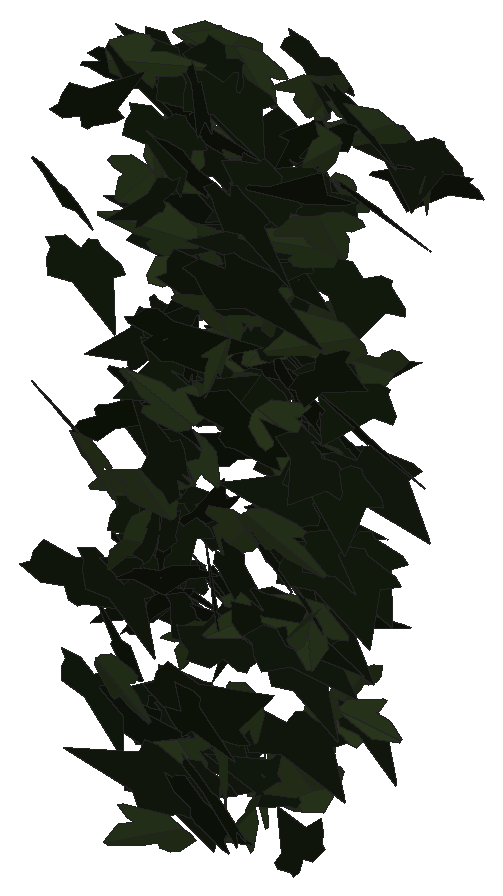
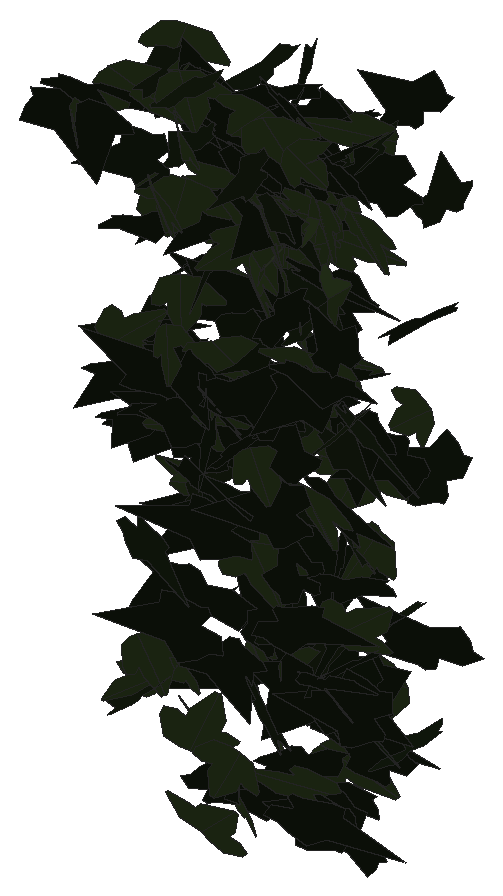
# SketchUp Ruby script. Lengths in millimetres.
U = 1.mm
M = Sketchup.active_model
def pt(a) = Geom::Point3d.new(a.map { |v| v * U })
def face(e, loops, mat)
  f = e.add_face(loops[0].map { |a| pt(a) })
  loops[1..].each { |l| e.add_face(l.map { |a| pt(a) }).erase! }
  f.material = f.back_material = mat if mat
  f
end
# faces: each face lists its corners as indices into pts; further lists are holes
def faces(e, pts, list, mat = nil) = list.each { |f| face(e, (f[0].is_a?(Array) ? f : [f]).map { |l| l.map { |i| pts[i] } }, mat) }
# xy, xz, yz: faces in a plane at the given z, y or x. An outline is a flat list of corners, or four numbers for a rectangle; further outlines are holes
def ring(l) = l.size == 4 ? [[l[0], l[1]], [l[2], l[1]], [l[2], l[3]], [l[0], l[3]]] : l.each_slice(2).to_a
def flat(e, list, mat, &to3) = list.each { |f| face(e, (f[0].is_a?(Array) ? f : [f]).map { |l| ring(l).map { |u, v| to3.(u, v) } }, mat) }
def xy(e, z, list, mat = nil) = flat(e, list, mat) { |x, y| [x, y, z] }
def xz(e, y, list, mat = nil) = flat(e, list, mat) { |x, z| [x, y, z] }
def yz(e, x, list, mat = nil) = flat(e, list, mat) { |y, z| [x, y, z] }
def lines(e, pts, list) = list.each { |a, b| e.add_line(pt(pts[a]), pt(pts[b])) }
# prism: a flat outline (further loops are holes) pulled along v
def prism(e, loops, v, mat = nil)
  f = face(e, loops, mat); d = Geom::Vector3d.new(v.map { |x| x * U })
  f.pushpull(f.normal.samedirection?(d) ? d.length : -d.length)
end
def box(e, o, s, mat = nil) = prism(e, [[o, [o[0] + s[0], o[1], o[2]], [o[0] + s[0], o[1] + s[1], o[2]], [o[0], o[1] + s[1], o[2]]]], [0, 0, s[2]], mat)
def at(x, y, z, deg = 0) = Geom::Transformation.translation(pt([x, y, z])) * Geom::Transformation.rotation(ORIGIN, Z_AXIS, deg.degrees)
def axes(o, x, y, z) = Geom::Transformation.new([*x, 0, *y, 0, *z, 0, *pt(o).to_a, 1])
def part(name) = M.definitions.add(name)
# library, detail: a bought-in or finely detailed component or shape, given as its bounding box
def library(name, o, s) = part(name).tap { |d| box(d.entities, o, s) }
def detail(e, o, s) = box(e.add_group.entities, o, s)
def put(e, d, t, mat = nil) = e.add_instance(d, t).tap { |i| i.material = mat if mat }
def group(e, t, mat = nil) = e.add_group.tap { |g| g.transformation = t; g.material = mat if mat }.entities
root = M.entities
M.materials.add("efeu1").color = [18, 25, 13]
M.materials.add("efeu2").color = [43, 57, 29]
c1 = part("ivyleaf_9")
p = [[39.1,54.8,31.7],[34.5,51.8,30.2],[-5.3,25.2,17.3],[-17.9,28.3,20.9],[-21.6,21.7,17],[-20.2,4.3,5.3],
  [-22.9,-0.3,2.5],[-17.1,-4,-0.6],[-2,-2.1,-1.2],[-0.7,-15.4,-10.1],[16.6,-22.3,-16.7],[21.1,-15.1,-12.5],
  [32.7,-10.7,-11],[46.1,-1.8,-6.6],[30.8,11.2,3.8]]
faces(c1.entities,p,[[0,1,2,3,4,5,6,7,8,9,10,11,12,13,14]],"efeu1")
c2 = part("ivyleaf_10")
p = [[0,12.8,-0.8],[-1.5,51.3,-10.9],[-4.9,51,-11.6],[-13.6,26.5,-7.3],[-13.2,15.9,-4.6],[-21.1,19.3,-7.2],
  [-29.5,16.3,-8.3],[-29.2,8.3,-6.2],[-19.7,-9.8,0.5],[-7.6,-13,4],[1,-12.2,5.8],[-0.4,51.1,-11.1],
  [-1.5,51.1,-10.9],[1,-12.4,5.9],[16.9,-12.4,3.5],[35.1,9.1,-5.1],[35,12.9,-6.1],[20.5,16.4,-4.9],
  [15.8,15,-3.8],[15.3,27.6,-7.1],[12.8,31.3,-7.8]]
faces(c2.entities,p,[[0,1,2,3,4,5,6,7,8,9,10],[11,12,0,13,14,15,16,17,18,19,20]],"efeu2")
put(root,c1,axes([4522.1,502.7,1812.9],[0.11464,-0.81055,1.02124],[0.40041,-1.00289,-0.80839],[2.44889,0.20192,0.08437]))
put(root,c2,axes([4486.9,625,1716.7],[-0.04389,0.08063,-1.16362],[-0.32409,-1.15161,-0.07642],[-2.19612,0.16833,0.03453]))
put(root,c1,axes([4401.2,621.1,1696.8],[0.38812,-0.35155,1.12904],[0.93477,-1.01702,-0.40539],[2.04723,0.53102,-0.02895]))
put(root,c2,axes([4248.1,609.8,2133.8],[-1.15954,0.6898,-0.52411],[0.68185,-0.38277,-0.92024],[-1.50119,-0.70666,-0.01315]))
put(root,c1,axes([4579.4,634.2,2221.9],[-0.57581,-0.81607,0.64489],[-0.44092,-0.60188,-0.87033],[1.92984,-0.38101,-0.00643]))
put(root,c1,axes([4456.5,626.9,2527],[0.99971,-1.1541,-0.11164],[-0.06222,0.10778,-1.26793],[2.20586,0.52608,0.01483]))
put(root,c1,axes([4356.1,616.6,2496.9],[-1.10006,0.89862,-0.10934],[0.11642,-0.09065,-1.06846],[-1.71893,-0.58123,-0.00239]))
put(root,c2,axes([4352.5,633.1,1646.7],[-0.9479,-0.4723,0.85777],[-1.24545,-0.55534,-0.68575],[1.38632,-0.82184,-0.02956]))
put(root,c1,axes([4181.7,643.5,2446.3],[1.299,-0.51553,-0.61479],[0.90646,-0.38921,0.85514],[-1.22883,-0.83207,-0.01909]))
put(root,c1,axes([4440.5,639.2,2420.9],[-0.18542,-0.10391,-1.25306],[2.02465,0.66316,-0.1377],[1.27564,-1.06764,0.03642]))
put(root,c1,axes([4430.4,649.4,2204.1],[0.45939,-0.11874,1.26812],[1.9734,-0.73122,-0.26583],[1.40771,1.06381,-0.04118]))
put(root,c1,axes([4349.9,647.2,1702.4],[-0.94184,-0.25561,-1.00449],[-1.71733,-0.44148,0.55688],[-0.97068,1.02908,-0.0106]))
put(root,c2,axes([4576.1,640.5,2534.3],[-1.459,-0.75984,-0.39655],[0.54037,0.27685,-1.07936],[1.53911,-0.81749,0.00305]))
put(root,c1,axes([4224.3,636.4,2558.9],[-0.19897,-0.20583,1.03103],[1.73227,0.5009,0.19229],[-1.00157,0.90722,0.12775]))
put(root,c2,axes([4409.7,660.9,2300.3],[1.23298,-1.01004,0.30154],[0.30524,-0.25537,-1.19995],[1.98278,0.6674,-0.00279]))
put(root,c2,axes([4552.6,662.3,2482.1],[-0.18039,-0.03356,1.07827],[-1.64646,-0.64432,-0.09609],[1.22664,-0.86977,0.02958]))
put(root,c1,axes([4403.4,650.2,2373.7],[-0.78734,-0.0999,1.16594],[2.20735,-0.19954,0.39442],[0.29632,1.22096,0.15985]))
put(root,c2,axes([4237.1,671.7,1801.6],[-0.73951,0.41482,-0.98164],[1.22992,-0.73911,-0.56813],[-1.61276,-0.75387,0.01685]))
put(root,c2,axes([4470.1,665.8,2081.6],[-1.1312,0.29702,-0.96008],[1.67524,-0.38438,-0.66385],[-0.92294,-1.06173,-0.02824]))
put(root,c2,axes([4493.4,648.7,2239.4],[0.52644,0.76003,0.69866],[0.30704,0.68259,-0.80643],[-1.94065,0.31417,0.06194]))
put(root,c2,axes([4349.8,661.1,2190.3],[0.97187,0.17477,0.90056],[-1.72236,-0.07277,0.52728],[0.28584,-1.0327,0.11525]))
put(root,c1,axes([4565.2,646.3,2329.4],[0.00954,-0.06713,-1.08285],[-0.68902,1.02069,-0.06495],[1.94649,0.36164,-0.01769]))
put(root,c1,axes([4151.4,685.2,2110.8],[0.98589,-0.87592,0.7521],[0.67161,-0.66475,-1.01725],[2.0921,0.62617,-0.02786]))
put(root,c1,axes([4473.1,661.1,2053.7],[1.49911,-0.39827,-0.60365],[-0.94481,0.35129,-0.87955],[1.00088,0.92813,0.07387]))
put(root,c1,axes([4309.7,668.6,2276.1],[1.94444,0.21551,-0.642],[0.98188,0.50504,0.99055],[0.8349,-1.09586,0.33025]))
put(root,c1,axes([4499.2,680.7,2452.1],[-1.57195,0.02987,0.6706],[-1.27733,-0.01689,-0.82588],[-0.02385,-1.06378,0.03195]))
put(root,c1,axes([4412.9,669.2,2015.6],[1.09499,-0.68369,-0.57412],[-0.67676,0.451,-0.89342],[1.55853,0.67618,0.01541]))
put(root,c2,axes([4516.5,680.5,1974.7],[2.17533,-0.24618,0.39364],[0.72898,-0.09114,-1.16917],[0.49938,1.20543,-0.008]))
put(root,c1,axes([4317,686.5,2507.8],[1.17099,-0.59217,0.85144],[1.12884,-0.61121,-0.8537],[1.6192,0.85437,-0.02059]))
put(root,c2,axes([4529,660.4,1958.8],[0.36015,-0.52337,0.92037],[-0.22603,0.91856,0.54676],[-2.00234,-0.19783,0.10382]))
put(root,c1,axes([4322.1,687.6,1788.8],[0.29318,-0.15283,-1.02701],[1.97602,0.01201,0.15395],[-0.0203,-1.03843,0.15293]))
put(root,c2,axes([4283.1,672.5,2076.7],[-1.83706,-0.68544,-0.45912],[0.69618,0.2778,-1.18378],[1.40735,-1.03215,-0.01371]))
put(root,c1,axes([4326.5,680,2090.2],[-0.49226,-1.05824,0.68082],[0.43762,0.6436,1.08774],[-2.35452,0.34087,0.05983]))
put(root,c1,axes([4450.4,677.8,1956.9],[0.27445,-0.06873,-1.20958],[1.87741,0.71386,0.07704],[1.33866,-0.98706,0.13994]))
put(root,c1,axes([4396.9,670.9,1930.6],[-0.08671,-0.39737,0.98233],[0.29014,0.97055,0.39967],[-1.99576,0.15836,0.01543]))
put(root,c1,axes([4457,703.8,2505.9],[-1.12715,-0.62701,0.63319],[-0.8485,-0.4498,-0.8624],[1.46844,-0.74119,-0.01229]))
put(root,c1,axes([4346.2,685.5,1779.4],[-0.51184,0.16016,1.1879],[1.85722,-0.67772,0.3123],[1.32474,1.012,0.02114]))
put(root,c2,axes([4555.9,698.1,2345.6],[-0.90612,-0.39925,1.03517],[-1.35145,-0.75588,-0.61812],[1.62247,-0.85259,0.06326]))
put(root,c1,axes([4296.9,698.5,2544.1],[-0.25525,-1.04425,-0.11183],[0.0261,0.11099,-1.05282],[1.9986,-0.13482,-0.00053]))
put(root,c2,axes([4444.9,701.2,1942.5],[1.06002,0.4708,-0.95349],[-1.3618,-0.63032,-0.72919],[-1.49715,0.90667,-0.01183]))
put(root,c1,axes([4309.2,676.1,1958.5],[0.90218,0.92692,-0.14562],[-0.16737,-0.11854,-1.04082],[-1.77789,0.48152,0.02409]))
put(root,c2,axes([4373.1,711.5,1711.5],[0.06809,-0.37054,1.19304],[1.39332,-0.96089,-0.32039],[1.92654,0.70804,0.18955]))
put(root,c1,axes([4554.9,695.8,2050.4],[-0.84814,-0.98323,-0.68623],[0.54736,0.62307,-1.0795],[2.21536,-0.53037,0.004]))
put(root,c1,axes([4492.5,685,1934.2],[-0.06895,-0.58858,-0.97281],[0.33301,0.95882,-0.58664],[2.13818,-0.16831,0.05999]))
put(root,c1,axes([4171,700.8,2325.9],[0.14105,-1.12983,-0.26375],[-0.0636,0.2621,-1.13215],[2.20718,0.07976,-0.01577]))
put(root,c1,axes([4333.6,715.4,2599.6],[0.46641,-0.3699,-1.06214],[1.60757,-0.65725,0.42378],[-1.41338,-0.86961,0.1315]))
put(root,c1,axes([4544.4,708.5,2155.6],[-0.51275,-1.14556,-0.1084],[0.04839,0.10538,-1.17682],[2.18944,-0.27061,0.00063]))
put(root,c2,axes([4379.4,692.9,2333.4],[-1.99212,-0.12524,-0.14372],[0.2731,0.01044,-1.05417],[0.23886,-1.05649,0.00662]))
put(root,c2,axes([4258.7,677.6,1985.2],[-0.40537,-0.66723,-1.05474],[0.61012,1.00485,-0.7004],[2.29563,-0.38488,-0.0001]))
put(root,c1,axes([4178.9,715.5,1752.8],[0.22527,-1.17167,0.39629],[0.16328,-0.38937,-1.17682],[2.34836,0.13947,0.04381]))
put(root,c2,axes([4429.1,694.6,1812.6],[1.23215,-0.81978,-0.44762],[-0.38254,0.40959,-1.04085],[1.73598,0.67211,0.08834]))
put(root,c1,axes([4516.7,680.6,1647.5],[-0.1238,0.55061,0.92319],[-0.3705,0.90356,-0.55261],[-2.01196,-0.20027,0.04495]))
put(root,c1,axes([4316.9,723.4,2203.1],[-1.08595,-0.59166,0.84111],[-1.076,-0.62302,-0.82178],[1.63487,-0.80305,0.01784]))
put(root,c1,axes([4154.9,695.2,1879.3],[-0.59379,0.09261,1.06489],[1.98427,-0.21825,0.32444],[0.44859,1.08798,-0.02556]))
put(root,c1,axes([4206.9,713.3,1910.3],[0.51131,-1.24201,-0.01926],[-0.00767,0.01883,-1.27073],[2.36406,0.26869,0.00004]))
put(root,c1,axes([4296,681.8,1985.6],[0.09494,0.51626,0.91873],[-0.2771,0.91432,-0.50587],[-1.98645,-0.10287,0.11447]))
put(root,c1,axes([4216.1,712.1,1715.9],[0.25318,-0.1585,1.03006],[1.29218,-0.77464,-0.20688],[1.50482,0.69185,0.00434]))
put(root,c1,axes([4463.9,720.2,2010.2],[0.46185,-1.05378,0.43407],[0.1756,-0.42418,-1.08135],[2.16192,0.25957,-0.0049]))
put(root,c2,axes([4306.8,710.1,2391.5],[-0.00778,0.02885,1.12319],[-1.94972,-0.46136,0.00812],[0.87817,-1.02407,0.02798]))
put(root,c1,axes([4244.6,697,1801.5],[0.11836,-0.48274,0.92118],[-0.31369,0.90659,0.48622],[-1.95432,-0.17475,-0.02225]))
put(root,c1,axes([4344.9,693.6,2305],[-0.68337,1.08501,0.13916],[-0.09392,0.13024,-1.14286],[-2.07978,-0.36239,0.00589]))
put(root,c1,axes([4469.2,710.4,2496.7],[1.8483,0.44547,0.31863],[-0.5464,-0.13833,1.06844],[0.88769,-1.01269,-0.00578]))
put(root,c1,axes([4562.8,711.1,2066.1],[-0.46002,-0.94463,-0.66097],[0.41125,0.62625,-0.97403],[2.15533,-0.32111,0.04478]))
put(root,c1,axes([4207.6,689,2124.3],[-0.06249,0.38685,-0.9635],[-0.14305,0.96056,0.38823],[1.97083,0.08199,-0.00237]))
put(root,c2,axes([4456.1,691.3,2353],[0.13169,-0.06917,-1.13677],[0.40142,1.11995,-0.05531],[2.13001,-0.20679,0.08071]))
put(root,c1,axes([4298.3,719.1,1668.3],[-1.06681,-0.56211,-0.83031],[1.24363,0.51672,-0.79094],[1.44743,-0.85826,0.06761]))
put(root,c1,axes([4287.5,703.1,1988.2],[0.38934,-0.17743,-1.01776],[-1.48134,0.65577,-0.27077],[1.29293,0.80477,-0.00375]))
put(root,c2,axes([4355.4,713.1,2180.9],[-1.58996,0.14601,0.82284],[-1.55423,0.10438,-0.84765],[-0.33767,-1.16794,0.02711]))
put(root,c1,axes([4321.6,712.7,2166.4],[-0.60372,-0.00406,1.00677],[1.91584,0.01593,0.31724],[-0.03124,1.05544,-0.00091]))
put(root,c1,axes([4372.9,714.7,1850.6],[-1.23796,-0.35059,0.76086],[1.27873,0.35705,0.73892],[-0.95234,0.93516,0.00312]))
put(root,c1,axes([4509.3,737.2,2508],[-1.68806,-0.494,0.0921],[-0.15898,-0.03928,-1.01523],[0.94307,-0.89086,-0.0063]))
put(root,c1,axes([4328.2,710.1,2221.4],[-0.16221,-0.32975,1.00135],[0.65364,0.94113,0.33915],[-1.89698,0.35248,0.03124]))
put(root,c1,axes([4357.9,731.2,2423.4],[-1.93424,0.07176,-0.20999],[0.40031,-0.00236,-1.01876],[-0.13466,-1.03777,-0.01221]))
put(root,c1,axes([4264.1,714,2162.6],[1.61297,0.1121,-0.95635],[-1.8258,-0.01119,-0.85146],[-0.1575,1.27779,0.07644]))
put(root,c2,axes([4276.2,707.4,2462.8],[0.04746,-0.41064,-0.96815],[0.12219,0.96721,-0.40859],[1.99774,-0.0494,0.04799]))
put(root,c1,axes([4304,722.1,2409.6],[0.8474,-0.1165,1.03505],[1.92409,-0.22256,-0.45994],[0.47706,1.10456,0.01649]))
put(root,c2,axes([4353.6,723.8,2401.4],[-1.93046,-0.36403,0.04194],[-0.07516,-0.01411,-1.07767],[0.69334,-1.01509,-0.00006]))
put(root,c2,axes([4278.8,728.7,2464],[1.93161,-0.42771,-0.4023],[0.70601,-0.15568,1.10137],[-0.86627,-1.0806,0.00056]))
put(root,c2,axes([4393.9,730.6,2400],[0.29455,-1.02543,-0.10195],[-0.03078,0.10066,-1.03704],[1.96098,0.15561,-0.00097]))
put(root,c2,axes([4240.6,727.8,2439.4],[1.51865,-0.52664,-0.39578],[-0.53731,0.28831,-0.95283],[1.13282,0.84276,0.07864]))
put(root,c1,axes([4454,732.9,1777.6],[-0.71926,-0.46471,-0.9378],[1.32705,0.63178,-0.59406],[1.48551,-0.78939,0.07662]))
put(root,c2,axes([4394.4,739.1,2324.8],[1.21568,-1.02807,0.04551],[0.03947,-0.04069,-1.21034],[1.95814,0.63908,-0.00386]))
put(root,c1,axes([4458.6,742.7,1862.6],[0.4071,-1.10488,-0.24681],[-0.0823,0.24302,-1.12539],[2.15307,0.2182,0.00365]))
put(root,c1,axes([4404.9,732,2394.6],[-0.28434,-0.23257,-1.00547],[1.03455,0.84586,-0.27642],[1.66958,-0.56374,0.00004]))
put(root,c1,axes([4460.9,761.6,2067],[-0.38813,-0.14405,1.19482],[-1.86085,-0.68673,-0.24968],[1.33544,-0.99879,-0.00065]))
put(root,c1,axes([4347.7,746.7,2590.4],[-0.23068,-0.97443,-0.49667],[0.30159,0.47879,-0.97802],[2.05957,-0.17925,0.08759]))
put(root,c2,axes([4373.8,764.1,2185.1],[0.08232,0.06862,-1.05561],[-1.16972,-0.85825,-0.08097],[-1.6386,0.61611,0.00477]))
put(root,c1,axes([4411.8,728.7,2457.2],[0.03788,-0.13283,1.13701],[0.88756,1.03948,0.11327],[-1.9897,0.46116,0.07217]))
put(root,c1,axes([4405.2,734.4,2273.7],[-0.74395,-0.25075,1.19291],[2.04131,0.52453,0.46171],[-1.1024,1.14048,0.04993]))
put(root,c2,axes([4463.1,761.9,1689.6],[-1.17363,-0.76684,-0.5738],[-0.69347,-0.44329,0.98402],[-1.68572,0.71625,-0.00531]))
put(root,c2,axes([4486.2,770.6,2546.3],[-0.25144,0.13974,1.10923],[0.5807,-1.07004,0.17114],[2.047,0.32072,0.0877]))
put(root,c1,axes([4281.4,773.9,1845.1],[-0.64236,-0.47663,1.00169],[-0.18657,-1.03012,-0.52318],[2.10297,-0.23698,0.25955]))
put(root,c1,axes([4255.9,749,2155.9],[-0.77562,0.83497,-0.34004],[0.25198,-0.31369,-0.92895],[-1.69723,-0.42815,0.01748]))
put(root,c1,axes([4240.7,759.3,1975.4],[-0.71528,-0.89923,-0.48626],[0.45426,0.42658,-0.97333],[1.89184,-0.44241,0.04986]))
put(root,c1,axes([4505.6,761.2,2200.7],[1.46786,-0.74947,0.54507],[0.73038,-0.38718,-1.07539],[1.60539,0.86141,-0.00912]))
put(root,c1,axes([4191.1,755.1,2574.9],[1.21647,-0.90924,-0.27198],[-0.29503,0.22348,-1.11142],[1.78197,0.6577,0.00165]))
put(root,c1,axes([4355.7,760.5,2196.4],[-1.14261,-0.48133,-0.70867],[1.21396,0.32653,-0.76214],[1.08839,-0.8695,0.10609]))
put(root,c2,axes([4304.5,762.6,1841.5],[-0.52437,-1.10426,0.25761],[-0.08926,-0.25378,-1.13801],[2.15621,-0.27905,0.01554]))
put(root,c2,axes([4258.7,761,1682.5],[1.42838,-0.12421,0.72321],[1.38279,-0.01921,-0.75729],[0.19575,1.04209,0.07224]))
put(root,c2,axes([4202.6,746.6,2575.5],[0.15791,0.05631,-1.11578],[1.98611,0.39557,0.09756],[0.75917,-1.0466,-0.02316]))
put(root,c1,axes([4314.5,775.8,1896.5],[0.43043,-0.7876,0.74488],[0.42032,-0.71148,-0.81935],[2.01989,0.31588,0.01177]))
put(root,c1,axes([4543.4,754.3,2149.3],[-0.14147,-0.79998,-0.96205],[0.48076,0.93431,-0.79643],[2.33226,-0.24112,0.10582]))
put(root,c1,axes([4282.9,747.1,2066.8],[-1.27176,0.17931,-0.96748],[-1.85494,0.03991,0.68057],[0.25706,1.17513,0.12451]))
put(root,c1,axes([4331.8,775.9,1875],[-0.05326,-0.17929,1.15073],[0.7248,-1.08919,-0.16044],[2.09463,0.37233,0.08478]))
put(root,c1,axes([4244.4,733.3,1860.4],[-0.41801,0.51256,-1.13394],[-0.92675,1.02425,0.5573],[2.17951,0.53383,0.01949]))
put(root,c1,axes([4273.5,767.8,2505.8],[1.04281,-0.47737,0.79131],[1.2994,-0.41089,-0.72063],[1.18536,0.87038,0.09381]))
put(root,c1,axes([4478.1,770.6,2565.7],[-0.07512,0.6301,-0.86428],[0.16967,-0.85992,-0.631],[-2.02855,-0.09526,-0.02077]))
put(root,c2,axes([4284.7,766.5,2076.3],[1.97465,-0.62532,-0.1728],[-0.26131,0.10691,-1.21124],[1.20675,1.04639,0.02048]))
put(root,c1,axes([4424.4,760.4,2521.2],[-0.68073,0.23247,1.0327],[-1.55695,0.63106,-0.4254],[-1.27851,-0.89228,-0.03181]))
put(root,c2,axes([4437.3,765.4,2122.5],[1.31202,0.09709,0.99761],[1.84014,0.25479,-0.69293],[-0.50291,1.18556,0.06722]))
put(root,c2,axes([4469.7,778,1791.7],[1.16896,-0.43975,0.62161],[0.99455,-0.33742,-0.75505],[1.05401,0.8061,0.02305]))
put(root,c1,axes([4269.9,779,2184.8],[0.6642,-1.02825,0.09986],[0.02974,-0.10014,-1.08573],[1.96595,0.34891,-0.01731]))
put(root,c2,axes([4295.6,758.2,2156.2],[-0.85267,-0.72054,-0.65323],[0.66205,0.55291,-0.84846],[1.72854,-0.56721,0.00274]))
put(root,c1,axes([4418.7,787.7,2183.5],[-0.10048,-0.18333,1.15102],[0.53211,-1.12055,-0.16565],[2.15346,0.26833,0.09464]))
put(root,c1,axes([4224.5,765.1,2199.6],[-1.40351,0.85299,0.01221],[-0.03099,0.00207,-1.12752],[-1.62328,-0.73755,0.01097]))
put(root,c1,axes([4322.1,777.4,2601.8],[-1.61683,0.18638,-0.52079],[0.95012,-0.15267,-0.86899],[-0.45334,-0.98469,0.03615]))
put(root,c1,axes([4514.5,787.3,2231.7],[-1.2374,-0.90154,0.15842],[-0.17025,-0.13081,-1.11152],[1.73376,-0.65628,0.00392]))
put(root,c1,axes([4521.9,784.4,2373.7],[-1.0413,-0.95922,-0.06143],[0.06613,0.0509,-1.10428],[1.82813,-0.54821,0.00496]))
put(root,c1,axes([4386.8,770.4,2012.4],[1.67992,-0.36713,0.45083],[0.8045,-0.15749,-0.95586],[0.75973,0.97856,0.01531]))
put(root,c1,axes([4287.8,776.3,2482.3],[1.21394,-1.0423,-0.19078],[-0.19735,0.16021,-1.22197],[2.00699,0.6462,-0.00477]))
put(root,c1,axes([4494.7,787.1,2135.5],[-0.83179,-0.97645,-0.02745],[0.02271,0.02474,-1.0698],[1.85898,-0.43721,0.00078]))
put(root,c2,axes([4400.8,774.2,2452.3],[-1.14159,0.10924,-0.86829],[1.6287,-0.14699,-0.60967],[-0.34841,-1.04504,-0.00501]))
put(root,c1,axes([4284,774.7,2378.3],[-1.31495,0.40119,0.58922],[-1.09708,0.16828,-0.79051],[-0.7981,-0.89232,0.11584]))
put(root,c1,axes([4287.7,771.1,1730.5],[-0.06173,-0.78656,-0.84268],[0.04499,0.84238,-0.78719],[2.19342,-0.03941,-0.00757]))
put(root,c1,axes([4442.8,793.7,2495.7],[0.23057,-0.89375,0.53404],[0.13973,-0.52897,-0.90193],[1.97658,0.14165,0.00146]))
put(root,c2,axes([4287.3,771.6,2195.1],[1.66572,0.18903,-0.49509],[0.871,0.21239,0.89012],[0.50858,-0.98286,0.09713]))
put(root,c2,axes([4361.8,797.1,1657.9],[0.90139,-0.64672,0.95066],[1.26943,-0.68294,-0.79689],[1.78243,0.81343,0.08678]))
put(root,c1,axes([4411.2,793.5,1653.4],[-0.22689,0.01372,1.05028],[-1.86637,-0.38015,-0.10635],[0.71619,-0.9863,0.05559]))
put(root,c1,axes([4352.8,790.5,1669.2],[-0.46575,-0.24105,-0.9004],[-1.02273,-0.72416,0.33992],[-1.44951,0.5884,0.04948]))
put(root,c1,axes([4431,782.6,1913.4],[-0.61826,-0.39276,-1.11955],[1.63043,0.7254,-0.50306],[1.56219,-0.91253,0.08196]))
put(root,c1,axes([4150.4,770.2,2543.7],[1.41341,0.21526,0.69483],[1.27481,0.18485,-0.77319],[-0.53986,1.00007,-0.00665]))
put(root,c2,axes([4334.4,792.4,2435.4],[0.0337,-1.05257,0.22896],[0.07029,-0.22827,-1.05223],[2.0489,0.02514,0.03233]))
put(root,c1,axes([4218.4,796,1840.8],[-0.08522,0.28385,-0.9545],[-0.35724,-0.94074,-0.27095],[-1.86125,0.16756,0.09571]))
put(root,c1,axes([4225.9,793.4,1665.4],[0.97171,-0.44577,0.91835],[1.43272,-0.52911,-0.67535],[1.31221,0.90779,0.05732]))
put(root,c2,axes([4259.7,780.8,1696.3],[0.14586,-0.07733,-1.08822],[2.0547,0.16241,0.06449],[0.29888,-1.07876,0.08772]))
put(root,c1,axes([4353.3,783.2,2268.5],[1.96648,-0.47011,-0.23639],[-0.41829,0.08772,-1.13512],[0.90991,1.05631,-0.01094]))
put(root,c2,axes([4351.8,787.2,1981.8],[-1.88068,-0.16084,0.47575],[-0.89407,-0.07516,-1.00117],[0.33788,-1.09415,-0.00116]))
put(root,c1,axes([4279.6,790.9,1969],[0.79845,0.74012,0.55673],[-0.75489,-0.40871,0.84224],[1.59279,-0.56472,0.12008]))
put(root,c1,axes([4408.7,768.4,2421.8],[0.11199,-0.00993,-1.16856],[-0.64505,1.1196,-0.02658],[2.12848,0.33983,0.05343]))
put(root,c1,axes([4259,802.4,2540.6],[-0.59353,-1.12062,-0.0585],[0.04114,-0.0667,1.16257],[-2.13528,0.31021,0.03866]))
put(root,c2,axes([4209.9,798.4,1937.2],[-1.37495,-0.18182,-0.67944],[-1.23279,-0.20757,0.74428],[-0.52164,0.96978,0.03192]))
put(root,c1,axes([4194.1,798.8,1675.8],[-0.36925,-0.09533,-1.1181],[2.10594,0.1725,-0.20671],[0.35526,-1.12162,0.06324]))
put(root,c2,axes([4255.8,809,2304.6],[0.9475,-0.5565,0.79807],[0.9452,-0.62553,-0.746],[1.59227,0.70247,-0.03206]))
put(root,c1,axes([4192.2,797.6,1902],[0.39831,-0.9545,-0.35769],[-0.07296,0.35752,-0.97649],[1.9386,0.20957,0.03674]))
put(root,c1,axes([4246.3,812.4,2337.3],[0.29489,-0.91076,0.43693],[0.15844,-0.42902,-0.9238],[1.91596,0.17565,0.00915]))
put(root,c1,axes([4441.6,799.6,2143.2],[0.52936,0.01888,-0.94334],[1.74859,0.21843,0.27527],[0.40873,-0.95893,0.04413]))
put(root,c2,axes([4454.4,795.4,2309.1],[-1.01652,-0.91102,-0.14357],[0.14481,0.12182,-1.05604],[1.74927,-0.53949,0.00399]))
put(root,c1,axes([4474.9,801.8,2595.8],[1.22051,-0.82247,-0.0609],[-0.08889,0.0408,-1.04287],[1.56709,0.64288,-0.01172]))
put(root,c2,axes([4329.2,804.5,2457.9],[1.36321,-0.79352,0.09931],[0.1226,-0.07563,-1.06898],[1.51706,0.71916,-0.00284]))
put(root,c1,axes([4204.2,795.5,2211.3],[0.94474,-0.78547,-0.56603],[-0.48084,0.50896,-0.92784],[1.77877,0.55476,0.04981]))
put(root,c1,axes([4264,789.7,1840.7],[2.04418,0.16301,-0.25278],[-0.47503,-0.04004,-1.08637],[-0.31944,1.10269,-0.00208]))
put(root,c2,axes([4246.2,798.6,2475.6],[-0.19754,-0.0993,-1.15253],[2.19557,-0.0946,-0.09574],[-0.16308,-1.15332,0.10708]))
put(root,c1,axes([4307.2,792.2,2198.2],[1.55386,0.00088,0.77181],[1.46788,-0.04313,-0.81582],[0.05517,1.12269,-0.03195]))
put(root,c2,axes([4387.5,807.1,2256.3],[1.60261,0.61318,-0.5629],[-0.90636,-0.3018,-1.04117],[-1.29927,0.96687,0.03199]))
put(root,c1,axes([4218.9,797.3,1841.7],[-1.31509,0.71685,0.04568],[-0.06201,0.03204,-0.99566],[-1.36568,-0.69175,0.00122]))
put(root,c2,axes([4526.8,812,2569.9],[-1.11558,-0.48213,0.86381],[-1.16916,-0.6096,-0.7571],[1.47572,-0.84743,0.05318]))
put(root,c1,axes([4405.6,791,2377.6],[0.96119,-0.45378,-0.89868],[-1.33344,0.56358,-0.67831],[1.37593,0.86317,-0.02957]))
put(root,c1,axes([4336.7,799.9,2507.8],[1.35731,-0.67532,-0.39492],[-0.55088,0.26869,-0.98217],[1.38325,0.76966,-0.00364]))
put(root,c2,axes([4248.1,803.1,2285.5],[1.85446,0.48063,0.2078],[0.35311,0.09361,-1.08648],[-0.93191,0.9919,0.00185]))
put(root,c1,axes([4214.9,812.5,2564.1],[-1.36234,0.02079,-0.74056],[1.40768,-0.03885,-0.71602],[-0.08065,-1.02923,0.01207]))
put(root,c2,axes([4234,796.9,2452.1],[-1.06414,0.7616,0.28988],[-0.39655,0.20626,-0.94379],[-1.49938,-0.59508,0.04387]))
put(root,c1,axes([4489.5,804.7,2472.9],[1.60931,-0.47929,0.22331],[0.43551,-0.048,-0.9695],[0.90722,0.87325,0.06928]))
put(root,c2,axes([4238.6,820,2489.6],[-0.31417,0.58169,-0.82619],[0.51858,-0.7805,-0.60397],[-1.8518,-0.31726,-0.02897]))
put(root,c2,axes([4327,811.1,2591.8],[-1.68339,0.17651,-0.46194],[0.74616,-0.32662,-0.8755],[-0.5736,-0.9429,0.2168]))
put(root,c1,axes([4509.6,804.1,1967],[-0.85721,0.94914,-0.14608],[0.1209,-0.13154,-1.05058],[-1.82366,-0.45486,-0.00099]))
put(root,c1,axes([4215.5,820.2,1877.3],[-1.63769,-0.3948,-0.10499],[0.1794,0.04632,-0.94674],[0.75651,-0.86564,-0.00277]))
put(root,c2,axes([4284.3,811.2,2469.4],[1.60202,0.0159,0.54691],[1.03027,0.12165,-0.8367],[-0.15134,0.99642,0.09342]))
put(root,c2,axes([4491.8,817,1824.6],[-0.73707,-1.02299,0.20415],[-0.12152,-0.19411,-1.09381],[1.98162,-0.39241,0.00886]))
put(root,c2,axes([4435.9,814.1,2596],[-1.04588,-0.90199,0.0654],[-0.0604,-0.05725,-1.05621],[1.72011,-0.55045,0.00268]))
put(root,c2,axes([4522.3,829.4,2234.2],[-0.61454,-0.39598,-0.93235],[-1.08173,-0.73918,0.51078],[-1.59576,0.65357,0.01281]))
put(root,c1,axes([4381.7,802.7,2014.2],[0.92859,0.12942,-0.95774],[1.09092,0.82505,0.4035],[1.48091,-0.68893,0.3033]))
put(root,c1,axes([4297.4,824.5,2140.3],[1.91725,-0.51988,0.29536],[-0.48249,0.15271,1.13347],[-1.03062,-1.03862,0.01882]))
put(root,c1,axes([4289.6,795.5,2063.6],[1.0832,0.28094,0.92733],[1.56349,0.43039,-0.63459],[-0.9779,0.99932,0.0126]))
put(root,c2,axes([4495.9,798.9,1775],[0.36449,0.53619,0.82078],[0.52446,0.77314,-0.56937],[-1.79067,0.33558,0.00031]))
put(root,c2,axes([4366.5,811.9,1714.1],[-1.78958,0.45231,-0.11184],[0.18461,-0.05635,-1.0434],[-0.86734,-0.94525,0.00868]))
put(root,c2,axes([4440.4,812.7,2452.4],[-1.94614,-0.28227,-0.10508],[0.19309,0.02737,-1.06081],[0.53974,-1.02758,0.00061]))
put(root,c1,axes([4488.7,827,1767],[0.42146,-1.02238,0.08636],[0.05234,-0.0824,-1.04605],[1.95203,0.22295,0.0094]))
put(root,c1,axes([4293.3,810.8,2480.7],[-0.68159,0.92104,-0.16784],[0.1067,-0.15828,-0.9882],[-1.7786,-0.36245,0.00503]))
put(root,c2,axes([4296.5,836.2,2405],[-0.44825,-0.22752,0.99468],[0.93151,-0.92092,-0.09475],[1.70398,0.44358,0.31346]))
put(root,c1,axes([4385.4,810,1857.3],[1.02599,0.2843,-0.86239],[-1.59443,-0.23116,-0.5999],[-0.66666,0.9904,0.10753]))
put(root,c1,axes([4401.1,824.6,2199.3],[-1.72672,0.33822,-0.45101],[0.79374,-0.17226,-0.96816],[-0.72187,-0.99843,0.01426]))
put(root,c1,axes([4566.4,828.8,2553.2],[-1.36159,-0.61995,-0.43145],[0.66698,0.25397,-0.94604],[1.27339,-0.79591,0.03419]))
put(root,c1,axes([4274,843.3,2357.1],[0.00352,-0.20098,-1.11062],[0.83658,-1.0228,0.18582],[-1.97846,-0.43285,0.0766]))
put(root,c1,axes([4294.3,814.5,2472.1],[1.83815,-0.05279,-0.27389],[-0.5206,0.01388,-0.96726],[0.10387,1.00381,-0.00103]))
put(root,c1,axes([4250.9,830.4,1695.5],[-0.31509,-0.18541,-1.08955],[-1.49674,-0.75432,0.24786],[-1.47793,0.80345,-0.01873]))
put(root,c1,axes([4147,828.2,1856.4],[1.49376,-0.54343,0.64876],[1.01576,-0.36884,-0.95464],[1.24998,0.94914,0.00047]))
put(root,c2,axes([4293.6,832.1,2592],[-1.25552,-0.67976,0.40464],[-0.32963,-0.38998,-0.9375],[1.46905,-0.66846,0.13546]))
put(root,c2,axes([4305,822.2,2463.1],[0.77396,-0.89437,-0.35702],[-0.20768,0.34226,-0.98168],[1.82097,0.41916,0.03978]))
put(root,c1,axes([4266.3,841.3,1948.4],[-0.36351,-0.22183,-0.99104],[-0.49994,-0.96331,0.26625],[-1.86705,0.30113,0.12166]))
put(root,c2,axes([4304.7,837.4,2412.7],[0.15623,-0.90941,0.49107],[0.28294,-0.4771,-0.90839],[1.94654,0.14234,0.09262]))
put(root,c1,axes([4331,831.5,2201.5],[1.32664,-0.06657,0.72988],[-1.36509,0.1451,0.69824],[-0.28674,-0.99878,0.05279]))
put(root,c1,axes([4408.3,846.5,2604.4],[-0.22841,-0.90622,0.54631],[0.26321,-0.55853,-0.89611],[1.9966,-0.03004,0.18063]))
put(root,c1,axes([4394,816.5,2062.8],[-1.60697,0.68941,0.28292],[0.41139,-0.18259,1.09004],[1.35729,0.87157,0.00457]))
put(root,c1,axes([4395.3,816.6,2155.3],[0.81283,-0.24428,-0.92315],[-1.51445,0.46801,-0.49199],[1.0047,0.90309,0.00525]))
put(root,c2,axes([4454.8,837.3,2448.7],[1.29766,-0.83053,0.233],[0.27459,-0.18302,-1.07455],[1.61857,0.69691,-0.00451]))
put(root,c1,axes([4440.6,823.1,2230.6],[0.81191,0.16061,-0.87581],[-1.64567,-0.15706,-0.44999],[-0.40446,0.96144,0.07279]))
put(root,c1,axes([4305.5,840.1,1826.4],[-1.33131,0.41779,-0.85188],[1.34454,-0.47716,-0.81412],[-1.20543,-0.99365,0.03277]))
put(root,c2,axes([4222.1,822.2,2501.8],[0.90646,-0.66587,-0.57347],[-0.33127,0.56788,-0.80394],[1.63936,0.48293,0.15464]))
put(root,c1,axes([4251.8,809.2,2251.8],[-0.07645,0.06913,-1.16094],[-0.6139,1.1154,0.07758],[2.12658,0.32448,-0.01934]))
put(root,c2,axes([4190.7,849.3,2415.3],[-0.42538,0.2623,-0.98467],[-0.24332,-1.00733,-0.23932],[-1.92406,0.0694,0.24796]))
put(root,c1,axes([4585.1,825.1,2518.3],[1.02178,0.79531,-0.56534],[-0.59877,-0.46971,-0.95956],[-1.75791,0.62227,-0.00176]))
put(root,c2,axes([4392.2,826.7,1620.6],[1.92153,-0.13683,0.58896],[-1.10801,0.08956,1.01882],[-0.31074,-1.16542,0.00914]))
put(root,c1,axes([4415.7,815.6,1879.6],[0.45345,0.54284,-0.87349],[0.70185,0.7919,0.59272],[1.82714,-0.43891,-0.0109]))
put(root,c1,axes([4177.1,848.1,2333.3],[0.01226,-0.28757,0.95768],[0.56555,-0.91388,-0.27642],[1.81707,0.28638,0.07957]))
put(root,c2,axes([4241.3,845.9,2580.7],[-0.27303,-0.8239,0.59513],[-0.02373,-0.59956,-0.83303],[1.9342,-0.12366,0.07379]))
put(root,c2,axes([4446.1,828.4,2260],[-0.2946,-0.98608,-0.33996],[0.12487,0.3338,-0.99808],[1.98118,-0.16767,0.01236]))
put(root,c2,axes([4311,836.5,2146.2],[-0.77843,-0.94121,0.11609],[-0.05307,-0.11444,-1.02605],[1.80411,-0.40947,0.01991]))
put(root,c2,axes([4342.2,819.6,2418.9],[-0.76713,-0.46862,-0.85608],[1.01902,0.66821,-0.61787],[1.55295,-0.66996,-0.01745]))
put(root,c1,axes([4341.7,854.7,2150.3],[-0.50664,-0.55305,0.78255],[-0.73555,-0.68124,-0.61292],[1.66885,-0.46816,-0.03257]))
put(root,c1,axes([4217,842.8,2297.1],[-1.48923,-0.51324,-0.4636],[0.78305,0.21725,-0.93496],[1.05805,-0.88318,0.03943]))
put(root,c1,axes([4442.8,828.7,2202.7],[-0.10525,0.02805,1.04957],[1.97975,-0.14123,0.05859],[0.2713,1.04149,-0.02032]))
put(root,c2,axes([4412.8,845.4,2547.2],[1.06899,-0.66441,0.50846],[0.7232,-0.34301,-0.86799],[1.41858,0.67554,0.05935]))
put(root,c2,axes([4578,840.8,2514.3],[0.56423,-0.93548,0.17038],[0.44263,-0.10171,-0.96313],[1.75473,0.32646,0.18817]))
